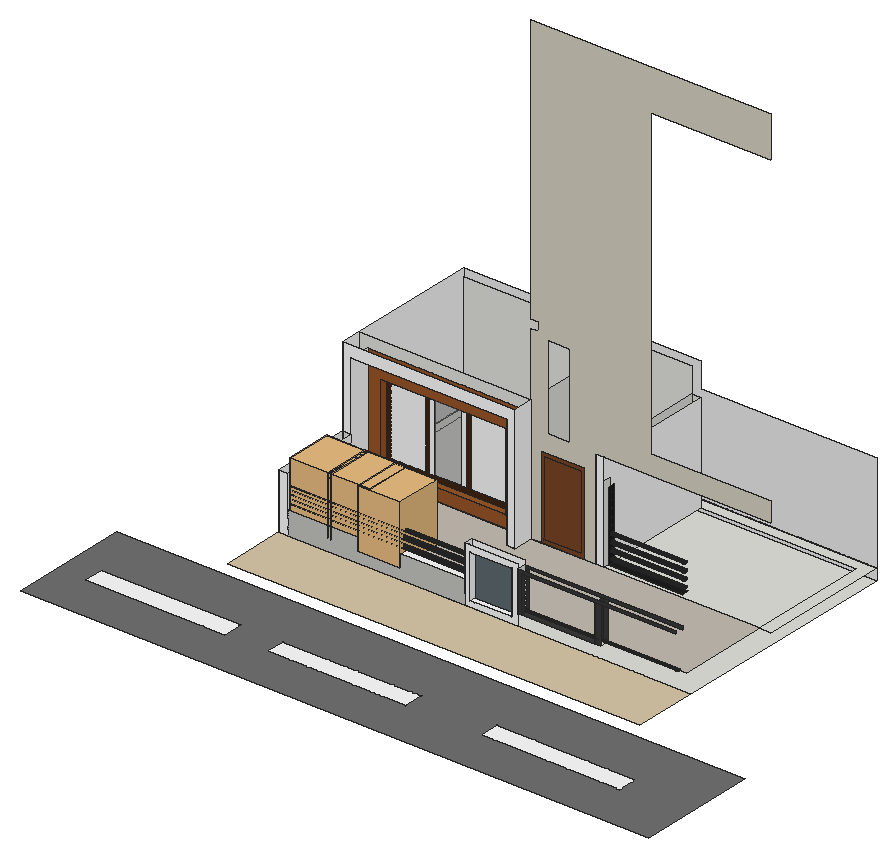
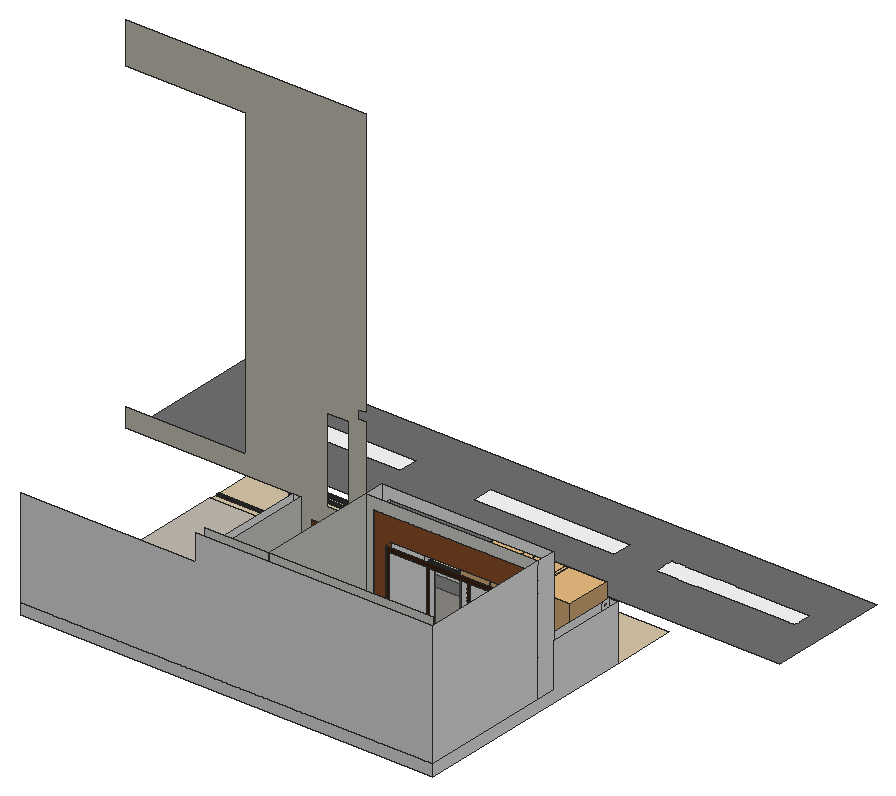
# SketchUp Ruby script. Lengths in inches.
U = 1.inch
M = Sketchup.active_model
def pt(a) = Geom::Point3d.new(a.map { |v| v * U })
def face(e, loops, mat)
  f = e.add_face(loops[0].map { |a| pt(a) })
  loops[1..].each { |l| e.add_face(l.map { |a| pt(a) }).erase! }
  f.material = f.back_material = mat if mat
  f
end
# faces: each face lists its corners as indices into pts; further lists are holes
def faces(e, pts, list, mat = nil) = list.each { |f| face(e, (f[0].is_a?(Array) ? f : [f]).map { |l| l.map { |i| pts[i] } }, mat) }
# xy, xz, yz: faces in a plane at the given z, y or x. An outline is a flat list of corners, or four numbers for a rectangle; further outlines are holes
def ring(l) = l.size == 4 ? [[l[0], l[1]], [l[2], l[1]], [l[2], l[3]], [l[0], l[3]]] : l.each_slice(2).to_a
def flat(e, list, mat, &to3) = list.each { |f| face(e, (f[0].is_a?(Array) ? f : [f]).map { |l| ring(l).map { |u, v| to3.(u, v) } }, mat) }
def xy(e, z, list, mat = nil) = flat(e, list, mat) { |x, y| [x, y, z] }
def xz(e, y, list, mat = nil) = flat(e, list, mat) { |x, z| [x, y, z] }
def yz(e, x, list, mat = nil) = flat(e, list, mat) { |y, z| [x, y, z] }
def lines(e, pts, list) = list.each { |a, b| e.add_line(pt(pts[a]), pt(pts[b])) }
# prism: a flat outline (further loops are holes) pulled along v
def prism(e, loops, v, mat = nil)
  f = face(e, loops, mat); d = Geom::Vector3d.new(v.map { |x| x * U })
  f.pushpull(f.normal.samedirection?(d) ? d.length : -d.length)
end
def box(e, o, s, mat = nil) = prism(e, [[o, [o[0] + s[0], o[1], o[2]], [o[0] + s[0], o[1] + s[1], o[2]], [o[0], o[1] + s[1], o[2]]]], [0, 0, s[2]], mat)
def at(x, y, z, deg = 0) = Geom::Transformation.translation(pt([x, y, z])) * Geom::Transformation.rotation(ORIGIN, Z_AXIS, deg.degrees)
def axes(o, x, y, z) = Geom::Transformation.new([*x, 0, *y, 0, *z, 0, *pt(o).to_a, 1])
def part(name) = M.definitions.add(name)
# library, detail: a bought-in or finely detailed component or shape, given as its bounding box
def library(name, o, s) = part(name).tap { |d| box(d.entities, o, s) }
def detail(e, o, s) = box(e.add_group.entities, o, s)
def put(e, d, t, mat = nil) = e.add_instance(d, t).tap { |i| i.material = mat if mat }
def group(e, t, mat = nil) = e.add_group.tap { |g| g.transformation = t; g.material = mat if mat }.entities
root = M.entities
M.materials.add("[Blinds Vertical Stripe Gray]").color = [247, 247, 247]
M.materials.add("[Carrera Marble]").color = [252, 252, 252]
M.materials.add("[Carrera Marble]1").color = [234, 234, 234]
M.materials.add("[Color M00]").color = [255, 255, 255]
M.materials.add("[Color M05]").color = [114, 114, 114]
M.materials.add("[Color M07]").color = [58, 58, 58]
M.materials.add("[Color M08]").color = [30, 30, 30]
M.materials.add("[Concrete Block 8x8 Gray]").color = [197, 198, 193]
M.materials.add("[Field Rectangle Tile]").color = [196, 189, 179]
M.materials.add("[Field Square Tile]").color = [217, 201, 169]
M.materials.add("[Formica Graystone]").color = [214, 209, 194]
M.materials.add("[Formica Laminate Dark]").color = [50, 53, 60]
M.materials.add("[Formica Speckled Grey]").color = [94, 105, 111]
M.materials.add("[Translucent Glass Gray]").color = [128, 128, 128]
M.materials["[Translucent Glass Gray]"].alpha = 0.5
M.materials.add("[Wood Cherry Original]").color = [152, 86, 42]
M.materials.add("[Wood Veneer 01]").color = [66, 38, 20]
M.materials.add("[Wood Veneer 01]1").color = [120, 70, 37]
c1 = library("chau cay",[-24.34,-109.24,0],[56.46,62.58,79.69])
xy(root,0,[[134.55,270.82,694.52,585.18]])
xy(root,0,[[39.61,61.99,228.17,88.8],[285.48,61.99,474.04,88.8],[576.23,61.99,764.79,88.8]],"[Color M00]")
xy(root,0,[[[0,0,853.75,163.125],[39.61,61.99,228.17,88.8],[285.48,61.99,474.04,88.8],[576.23,61.99,764.79,88.8]]],"[Color M05]")
xy(root,0,[[134.55,183.4,694.52,270.82]],"[Field Square Tile]")
xy(root,7.93,[[394.4,270.82,451.35,278.69]],"[Carrera Marble]")
xy(root,15.1875,[[459.28,270.82,464.36,283.23],[564.04,270.82,571.61,283.23],[134.55,378.85,146.33,406.29],[357.05,378.85,369,406.29],[134.55,406.29,134.55,585.18,694.52,585.18,694.52,406.29,679.23,406.29,679.23,570.65,146.33,570.65,146.33,406.29],
  [146.33,406.29,369,570.65],[369,406.29,456.06,570.65],[456.06,406.29,467.61,570.65]])
xy(root,15.1875,[[464.36,270.82,564.04,283.23]],"[Color M07]")
xy(root,15.1875,[[146.33,283.23,679.23,283.23,679.23,406.29,369,406.29,369,378.85,357.05,378.85,357.05,406.29,146.33,406.29]],"[Field Rectangle Tile]")
xy(root,19.3125,[[473.77,406.29,574.36,416.16]],"[Color M08]")
xy(root,31.3125,[[146.33,270.82,386.47,283.23]],"[Carrera Marble]")
xy(root,31.93,[[163.95,406.29,333.85,416.16]],"[Wood Cherry Original]")
xz(root,270.82,[[134.55,0,146.33,75.25],[[386.47,0,459.28,75.25],[394.4,7.93,451.35,67.32]]],"[Carrera Marble]")
xz(root,270.82,[[459.28,15.1875,464.36,15.1875,464.36,65.34,673.42,65.34,673.42,69.375,459.28,69.375],[564.04,15.1875,571.61,65.34]],"[Color M07]")
xz(root,270.82,[[146.33,0,386.47,31.3125]],"[Concrete Block 8x8 Gray]")
xz(root,278.69,[[394.4,7.93,451.35,67.32]],"[Formica Speckled Grey]")
xz(root,283.23,[[386.47,15.1875,459.28,75.25]],"[Carrera Marble]")
xz(root,283.23,[[459.28,15.1875,459.28,69.375,673.42,69.375,673.42,65.34,464.36,65.34,464.36,15.1875],[564.04,15.1875,571.61,65.34]],"[Color M07]")
xz(root,283.23,[[146.33,15.1875,386.47,31.3125]],"[Concrete Block 8x8 Gray]")
xz(root,378.85,[[134.55,15.1875,146.33,75.25]])
xz(root,378.85,[[357.05,15.1875,369,15.1875,369,183.6875,134.55,183.6875,134.55,75.25,146.33,75.25,146.33,168.73,357.05,168.73]],"[Carrera Marble]")
xz(root,406.29,[[134.55,15.1875,134.55,183.6875,369,183.6875,369,15.1875,357.05,15.1875,357.05,168.73,146.33,168.73,146.33,15.1875]])
xz(root,406.29,[[456.06,15.1875,467.61,149.125]],"[Carrera Marble]")
xz(root,406.29,[[[369,15.1875,381.33,15.1875,381.33,126.53,442.15,126.53,442.15,15.1875,456.06,15.1875,456.06,149.125,694.52,149.125,694.52,175.14,531.06,175.14,531.06,590.25,694.52,590.25,694.52,645.75,369,645.75,369,282.625,378.87,282.625,378.87,270.8125,369,270.8125],[391.83,149.97,420.7,264.27]]],"[Formica Graystone]")
xz(root,406.29,[[[146.33,15.1875,357.05,168.73],[163.95,31.93,333.85,136.93]]],"[Wood Cherry Original]")
xz(root,406.29,[[[381.33,15.1875,442.15,126.53],[386.24,20.1,437.24,121.625]],[386.24,20.1,437.24,121.625]],"[Wood Veneer 01]1")
xz(root,416.16,[[170.57,38.55,217.46,130.31],[223.37,38.55,229.51,130.31],[266.3,38.55,272.95,130.31],[278.86,38.55,327.23,130.31]],"[Blinds Vertical Stripe Gray]")
xz(root,416.16,[[229.51,38.55,266.3,130.31]],"[Translucent Glass Gray]")
xz(root,416.16,[[[163.95,31.93,333.85,136.93],[170.57,38.55,327.23,130.31]],[217.46,38.55,223.37,130.31],[272.95,38.55,278.86,130.31]],"[Wood Veneer 01]")
xz(root,570.65,[[146.33,15.1875,369,183.6875],[369,15.1875,456.06,183.6875],[456.06,15.1875,467.61,149.125]])
xz(root,585.18,[[134.55,0,694.52,15.1875],[134.55,15.1875,134.55,183.6875,456.06,183.6875,456.06,149.125,694.52,149.125,694.52,15.1875]],"[Carrera Marble]1")
yz(root,134.55,[[270.82,0,270.82,75.25,378.85,75.25,378.85,15.1875,585.18,15.1875,585.18,0],[378.85,15.1875,406.29,183.6875],[406.29,15.1875,585.18,183.6875]],"[Carrera Marble]")
yz(root,146.33,[[277.43,35.26,276.8,35.35,276.21,35.59,275.71,35.98,275.32,36.48,275.08,37.07,274.99,37.7,275.08,38.33,275.32,38.92,275.71,39.42,276.21,39.8125,276.8,40.05,277.43,40.14,278.0625,40.05,278.65,39.8125,279.15,39.42,279.54,38.92,279.78,38.33,279.87,37.7,279.78,37.07,279.54,36.48,279.15,35.98,278.65,35.59,278.0625,35.35],[277.43,46.33,276.8,46.41,276.21,46.65,275.71,47.04,275.32,47.54,275.08,48.13,274.99,48.76,275.08,49.39,275.32,49.98,275.71,50.49,276.21,50.875,276.8,51.12,277.43,51.2,278.0625,51.12,278.65,50.875,279.15,50.49,279.54,49.98,279.78,49.39,279.87,48.76,279.78,48.13,279.54,47.54,279.15,47.04,278.65,46.65,278.0625,46.41],[277.43,57.01,276.8,57.1,276.21,57.34,275.71,57.73,275.32,58.23,275.08,58.82,274.99,59.45,275.08,60.08,275.32,60.67,275.71,61.17,276.21,61.5625,276.8,61.8,277.43,61.89,278.0625,61.8,278.65,61.5625,279.15,61.17,279.54,60.67,279.78,60.08,279.87,59.45,279.78,58.82,279.54,58.23,279.15,57.73,278.65,57.34,278.0625,57.1]])
yz(root,146.33,[[283.23,15.1875,378.85,75.25],[378.85,15.1875,406.29,168.73],[[270.82,31.3125,283.23,75.25],[277.43,35.26,276.8,35.35,276.21,35.59,275.71,35.98,275.32,36.48,275.08,37.07,274.99,37.7,275.08,38.33,275.32,38.92,275.71,39.42,276.21,39.8125,276.8,40.05,277.43,40.14,278.0625,40.05,278.65,39.8125,279.15,39.42,279.54,38.92,279.78,38.33,279.87,37.7,279.78,37.07,279.54,36.48,279.15,35.98,278.65,35.59,278.0625,35.35],[277.43,57.01,276.8,57.1,276.21,57.34,275.71,57.73,275.32,58.23,275.08,58.82,274.99,59.45,275.08,60.08,275.32,60.67,275.71,61.17,276.21,61.5625,276.8,61.8,277.43,61.89,278.0625,61.8,278.65,61.5625,279.15,61.17,279.54,60.67,279.78,60.08,279.87,59.45,279.78,58.82,279.54,58.23,279.15,57.73,278.65,57.34,278.0625,57.1],[277.43,46.33,276.8,46.41,276.21,46.65,275.71,47.04,275.32,47.54,275.08,48.13,274.99,48.76,275.08,49.39,275.32,49.98,275.71,50.49,276.21,50.875,276.8,51.12,277.43,51.2,278.0625,51.12,278.65,50.875,279.15,50.49,279.54,49.98,279.78,49.39,279.87,48.76,279.78,48.13,279.54,47.54,279.15,47.04,278.65,46.65,278.0625,46.41],[277.43,67.33,276.8,67.41,276.21,67.65,275.71,68.04,275.32,68.54,275.08,69.13,274.99,69.76,275.08,70.39,275.32,70.98,275.71,71.49,276.21,71.875,276.8,72.12,277.43,72.2,278.0625,72.12,278.65,71.875,279.15,71.49,279.54,70.98,279.78,70.39,279.87,69.76,279.78,69.13,279.54,68.54,279.15,68.04,278.65,67.65,278.0625,67.41]]],"[Carrera Marble]")
yz(root,163.95,[[406.29,31.93,416.16,136.93]],"[Wood Cherry Original]")
yz(root,333.85,[[406.29,31.93,416.16,136.93]],"[Wood Cherry Original]")
yz(root,357.05,[[378.85,15.1875,406.29,168.73]],"[Carrera Marble]")
yz(root,369,[[406.29,15.1875,570.65,183.6875]])
yz(root,369,[[378.85,15.1875,406.29,183.6875]],"[Carrera Marble]")
yz(root,386.47,[[270.82,15.1875,283.23,31.3125]])
yz(root,386.47,[[[270.82,31.3125,283.23,75.25],[277.43,67.33,278.0625,67.41,278.65,67.65,279.15,68.04,279.54,68.54,279.78,69.13,279.87,69.76,279.78,70.39,279.54,70.98,279.15,71.49,278.65,71.875,278.0625,72.12,277.43,72.2,276.8,72.12,276.21,71.875,275.71,71.49,275.32,70.98,275.08,70.39,274.99,69.76,275.08,69.13,275.32,68.54,275.71,68.04,276.21,67.65,276.8,67.41],[277.43,57.01,278.0625,57.1,278.65,57.34,279.15,57.73,279.54,58.23,279.78,58.82,279.87,59.45,279.78,60.08,279.54,60.67,279.15,61.17,278.65,61.5625,278.0625,61.8,277.43,61.89,276.8,61.8,276.21,61.5625,275.71,61.17,275.32,60.67,275.08,60.08,274.99,59.45,275.08,58.82,275.32,58.23,275.71,57.73,276.21,57.34,276.8,57.1],[277.43,46.33,278.0625,46.41,278.65,46.65,279.15,47.04,279.54,47.54,279.78,48.13,279.87,48.76,279.78,49.39,279.54,49.98,279.15,50.49,278.65,50.875,278.0625,51.12,277.43,51.2,276.8,51.12,276.21,50.875,275.71,50.49,275.32,49.98,275.08,49.39,274.99,48.76,275.08,48.13,275.32,47.54,275.71,47.04,276.21,46.65,276.8,46.41],[277.43,35.26,278.0625,35.35,278.65,35.59,279.15,35.98,279.54,36.48,279.78,37.07,279.87,37.7,279.78,38.33,279.54,38.92,279.15,39.42,278.65,39.8125,278.0625,40.05,277.43,40.14,276.8,40.05,276.21,39.8125,275.71,39.42,275.32,38.92,275.08,38.33,274.99,37.7,275.08,37.07,275.32,36.48,275.71,35.98,276.21,35.59,276.8,35.35]]],"[Carrera Marble]")
yz(root,394.4,[[270.82,7.93,278.69,67.32]],"[Carrera Marble]")
yz(root,451.35,[[270.82,7.93,278.69,67.32]],"[Carrera Marble]")
yz(root,456.06,[[406.29,15.1875,570.65,149.125]])
yz(root,459.28,[[270.82,15.1875,283.23,69.375]])
yz(root,464.36,[[276.43,17.77,276.06,17.82,275.71,17.96,275.41,18.1875,275.18,18.49,275.04,18.83,274.99,19.2,275.04,19.58,275.18,19.92,275.41,20.22,275.71,20.45,276.06,20.59,276.43,20.64,276.8,20.59,277.15,20.45,277.44,20.22,277.67,19.92,277.82,19.58,277.87,19.2,277.82,18.83,277.67,18.49,277.44,18.1875,277.15,17.96,276.8,17.82],[276.43,23.27,276.06,23.32,275.71,23.46,275.41,23.6875,275.18,23.99,275.04,24.33,274.99,24.7,275.04,25.08,275.18,25.42,275.41,25.72,275.71,25.95,276.06,26.09,276.43,26.14,276.8,26.09,277.15,25.95,277.44,25.72,277.67,25.42,277.82,25.08,277.87,24.7,277.82,24.33,277.67,23.99,277.44,23.6875,277.15,23.46,276.8,23.32],[276.43,28.77,276.06,28.82,275.71,28.96,275.41,29.1875,275.18,29.49,275.04,29.83,274.99,30.2,275.04,30.58,275.18,30.92,275.41,31.22,275.71,31.45,276.06,31.59,276.43,31.64,276.8,31.59,277.15,31.45,277.44,31.22,277.67,30.92,277.82,30.58,277.87,30.2,277.82,29.83,277.67,29.49,277.44,29.1875,277.15,28.96,276.8,28.82],[276.43,35.2,276.06,35.25,275.71,35.4,275.41,35.625,275.18,35.92,275.04,36.27,274.99,36.64,275.04,37.01,275.18,37.36,275.41,37.66,275.71,37.89,276.06,38.03,276.43,38.08,276.8,38.03,277.15,37.89,277.44,37.66,277.67,37.36,277.82,37.01,277.87,36.64,277.82,36.27,277.67,35.92,277.44,35.625,277.15,35.4,276.8,35.25],[276.43,41.89,276.06,41.94,275.71,42.08,275.41,42.3125,275.18,42.61,275.04,42.96,274.99,43.33,275.04,43.7,275.18,44.05,275.41,44.35,275.71,44.57,276.06,44.72,276.43,44.77,276.8,44.72,277.15,44.57,277.44,44.35,277.67,44.05,277.82,43.7,277.87,43.33,277.82,42.96,277.67,42.61,277.44,42.3125,277.15,42.08,276.8,41.94],
  [276.43,48.08,276.06,48.13,275.71,48.27,275.41,48.5,275.18,48.8,275.04,49.14,274.99,49.52,275.04,49.89,275.18,50.24,275.41,50.53,275.71,50.76,276.06,50.9,276.43,50.95,276.8,50.9,277.15,50.76,277.44,50.53,277.67,50.24,277.82,49.89,277.87,49.52,277.82,49.14,277.67,48.8,277.44,48.5,277.15,48.27,276.8,48.13],[276.43,53.89,276.06,53.94,275.71,54.08,275.41,54.3125,275.18,54.61,275.04,54.96,274.99,55.33,275.04,55.7,275.18,56.05,275.41,56.35,275.71,56.57,276.06,56.72,276.43,56.77,276.8,56.72,277.15,56.57,277.44,56.35,277.67,56.05,277.82,55.7,277.87,55.33,277.82,54.96,277.67,54.61,277.44,54.3125,277.15,54.08,276.8,53.94]])
yz(root,464.36,[[[270.82,15.1875,283.23,65.34],[276.43,17.77,276.06,17.82,275.71,17.96,275.41,18.1875,275.18,18.49,275.04,18.83,274.99,19.2,275.04,19.58,275.18,19.92,275.41,20.22,275.71,20.45,276.06,20.59,276.43,20.64,276.8,20.59,277.15,20.45,277.44,20.22,277.67,19.92,277.82,19.58,277.87,19.2,277.82,18.83,277.67,18.49,277.44,18.1875,277.15,17.96,276.8,17.82],[276.43,23.27,276.06,23.32,275.71,23.46,275.41,23.6875,275.18,23.99,275.04,24.33,274.99,24.7,275.04,25.08,275.18,25.42,275.41,25.72,275.71,25.95,276.06,26.09,276.43,26.14,276.8,26.09,277.15,25.95,277.44,25.72,277.67,25.42,277.82,25.08,277.87,24.7,277.82,24.33,277.67,23.99,277.44,23.6875,277.15,23.46,276.8,23.32],[276.43,48.08,276.06,48.13,275.71,48.27,275.41,48.5,275.18,48.8,275.04,49.14,274.99,49.52,275.04,49.89,275.18,50.24,275.41,50.53,275.71,50.76,276.06,50.9,276.43,50.95,276.8,50.9,277.15,50.76,277.44,50.53,277.67,50.24,277.82,49.89,277.87,49.52,277.82,49.14,277.67,48.8,277.44,48.5,277.15,48.27,276.8,48.13],[276.43,28.77,276.06,28.82,275.71,28.96,275.41,29.1875,275.18,29.49,275.04,29.83,274.99,30.2,275.04,30.58,275.18,30.92,275.41,31.22,275.71,31.45,276.06,31.59,276.43,31.64,276.8,31.59,277.15,31.45,277.44,31.22,277.67,30.92,277.82,30.58,277.87,30.2,277.82,29.83,277.67,29.49,277.44,29.1875,277.15,28.96,276.8,28.82],[276.43,41.89,276.06,41.94,275.71,42.08,275.41,42.3125,275.18,42.61,275.04,42.96,274.99,43.33,275.04,43.7,275.18,44.05,275.41,44.35,275.71,44.57,276.06,44.72,276.43,44.77,276.8,44.72,277.15,44.57,277.44,44.35,277.67,44.05,277.82,43.7,277.87,43.33,277.82,42.96,277.67,42.61,277.44,42.3125,277.15,42.08,276.8,41.94],[276.43,35.2,276.06,35.25,275.71,35.4,275.41,35.625,275.18,35.92,275.04,36.27,274.99,36.64,275.04,37.01,275.18,37.36,275.41,37.66,275.71,37.89,276.06,38.03,276.43,38.08,276.8,38.03,277.15,37.89,277.44,37.66,277.67,37.36,277.82,37.01,277.87,36.64,277.82,36.27,277.67,35.92,277.44,35.625,277.15,35.4,276.8,35.25],[276.43,59.2,276.06,59.25,275.71,59.4,275.41,59.625,275.18,59.92,275.04,60.27,274.99,60.64,275.04,61.01,275.18,61.36,275.41,61.66,275.71,61.89,276.06,62.03,276.43,62.08,276.8,62.03,277.15,61.89,277.44,61.66,277.67,61.36,277.82,61.01,277.87,60.64,277.82,60.27,277.67,59.92,277.44,59.625,277.15,59.4,276.8,59.25],[276.43,53.89,276.06,53.94,275.71,54.08,275.41,54.3125,275.18,54.61,275.04,54.96,274.99,55.33,275.04,55.7,275.18,56.05,275.41,56.35,275.71,56.57,276.06,56.72,276.43,56.77,276.8,56.72,277.15,56.57,277.44,56.35,277.67,56.05,277.82,55.7,277.87,55.33,277.82,54.96,277.67,54.61,277.44,54.3125,277.15,54.08,276.8,53.94]]],"[Color M07]")
yz(root,467.61,[[406.29,15.1875,416.16,119.75]])
yz(root,467.61,[[416.16,15.1875,570.65,15.1875,570.65,149.125,406.29,149.125,406.29,119.75,416.16,119.75]],"[Carrera Marble]")
yz(root,473.77,[[411.5,23.75,411,23.8125,410.53,24.01,410.13,24.32,409.82,24.72,409.63,25.18,409.5625,25.6875,409.63,26.1875,409.82,26.65,410.13,27.06,410.53,27.36,411,27.56,411.5,27.625,412,27.56,412.47,27.36,412.87,27.06,413.18,26.65,413.37,26.1875,413.4375,25.6875,413.37,25.18,413.18,24.72,412.87,24.32,412.47,24.01,412,23.8125],[411.5,33.75,411,33.8125,410.53,34.01,410.13,34.32,409.82,34.72,409.63,35.18,409.5625,35.6875,409.63,36.1875,409.82,36.65,410.13,37.06,410.53,37.36,411,37.56,411.5,37.625,412,37.56,412.47,37.36,412.87,37.06,413.18,36.65,413.37,36.1875,413.4375,35.6875,413.37,35.18,413.18,34.72,412.87,34.32,412.47,34.01,412,33.8125],[411.5,43.75,411,43.8125,410.53,44.01,410.13,44.32,409.82,44.72,409.63,45.18,409.5625,45.6875,409.63,46.1875,409.82,46.65,410.13,47.06,410.53,47.36,411,47.56,411.5,47.625,412,47.56,412.47,47.36,412.87,47.06,413.18,46.65,413.37,46.1875,413.4375,45.6875,413.37,45.18,413.18,44.72,412.87,44.32,412.47,44.01,412,43.8125],[411.5,53.75,411,53.8125,410.53,54.01,410.13,54.32,409.82,54.72,409.63,55.18,409.5625,55.6875,409.63,56.1875,409.82,56.65,410.13,57.06,410.53,57.36,411,57.56,411.5,57.625,412,57.56,412.47,57.36,412.87,57.06,413.18,56.65,413.37,56.1875,413.4375,55.6875,413.37,55.18,413.18,54.72,412.87,54.32,412.47,54.01,412,53.8125]])
yz(root,473.77,[[[406.29,19.3125,416.16,113.6],[411.5,83.75,411,83.8125,410.53,84.01,410.13,84.32,409.82,84.72,409.63,85.18,409.5625,85.6875,409.63,86.1875,409.82,86.65,410.13,87.06,410.53,87.36,411,87.56,411.5,87.625,412,87.56,412.47,87.36,412.87,87.06,413.18,86.65,413.37,86.1875,413.4375,85.6875,413.37,85.18,413.18,84.72,412.87,84.32,412.47,84.01,412,83.8125],[411.5,73.75,411,73.8125,410.53,74.01,410.13,74.32,409.82,74.72,409.63,75.18,409.5625,75.6875,409.63,76.1875,409.82,76.65,410.13,77.06,410.53,77.36,411,77.56,411.5,77.625,412,77.56,412.47,77.36,412.87,77.06,413.18,76.65,413.37,76.1875,413.4375,75.6875,413.37,75.18,413.18,74.72,412.87,74.32,412.47,74.01,412,73.8125],[411.5,63.75,411,63.8125,410.53,64.01,410.13,64.32,409.82,64.72,409.63,65.18,409.5625,65.6875,409.63,66.1875,409.82,66.65,410.13,67.06,410.53,67.36,411,67.56,411.5,67.625,412,67.56,412.47,67.36,412.87,67.06,413.18,66.65,413.37,66.1875,413.4375,65.6875,413.37,65.18,413.18,64.72,412.87,64.32,412.47,64.01,412,63.8125],[411.5,53.75,411,53.8125,410.53,54.01,410.13,54.32,409.82,54.72,409.63,55.18,409.5625,55.6875,409.63,56.1875,409.82,56.65,410.13,57.06,410.53,57.36,411,57.56,411.5,57.625,412,57.56,412.47,57.36,412.87,57.06,413.18,56.65,413.37,56.1875,413.4375,55.6875,413.37,55.18,413.18,54.72,412.87,54.32,412.47,54.01,412,53.8125],[411.5,43.75,411,43.8125,410.53,44.01,410.13,44.32,409.82,44.72,409.63,45.18,409.5625,45.6875,409.63,46.1875,409.82,46.65,410.13,47.06,410.53,47.36,411,47.56,411.5,47.625,412,47.56,412.47,47.36,412.87,47.06,413.18,46.65,413.37,46.1875,413.4375,45.6875,413.37,45.18,413.18,44.72,412.87,44.32,412.47,44.01,412,43.8125],[411.5,33.75,411,33.8125,410.53,34.01,410.13,34.32,409.82,34.72,409.63,35.18,409.5625,35.6875,409.63,36.1875,409.82,36.65,410.13,37.06,410.53,37.36,411,37.56,411.5,37.625,412,37.56,412.47,37.36,412.87,37.06,413.18,36.65,413.37,36.1875,413.4375,35.6875,413.37,35.18,413.18,34.72,412.87,34.32,412.47,34.01,412,33.8125],[411.5,23.75,411,23.8125,410.53,24.01,410.13,24.32,409.82,24.72,409.63,25.18,409.5625,25.6875,409.63,26.1875,409.82,26.65,410.13,27.06,410.53,27.36,411,27.56,411.5,27.625,412,27.56,412.47,27.36,412.87,27.06,413.18,26.65,413.37,26.1875,413.4375,25.6875,413.37,25.18,413.18,24.72,412.87,24.32,412.47,24.01,412,23.8125],[411.5,103.75,411,103.8125,410.53,104.01,410.13,104.32,409.82,104.72,409.63,105.18,409.5625,105.6875,409.63,106.1875,409.82,106.65,410.13,107.06,410.53,107.36,411,107.56,411.5,107.625,412,107.56,412.47,107.36,412.87,107.06,413.18,106.65,413.37,106.1875,413.4375,105.6875,413.37,105.18,413.18,104.72,412.87,104.32,412.47,104.01,412,103.8125],[411.5,93.75,411,93.8125,410.53,94.01,410.13,94.32,409.82,94.72,409.63,95.18,409.5625,95.6875,409.63,96.1875,409.82,96.65,410.13,97.06,410.53,97.36,411,97.56,411.5,97.625,412,97.56,412.47,97.36,412.87,97.06,413.18,96.65,413.37,96.1875,413.4375,95.6875,413.37,95.18,413.18,94.72,412.87,94.32,412.47,94.01,412,93.8125]]],"[Color M08]")
yz(root,564.04,[[270.82,15.1875,283.23,65.34]],"[Color M07]")
p = [[464.36,275.71,17.96],[464.36,276.06,17.82],[673.42,276.06,17.82],[673.42,275.71,17.96],[464.36,276.43,17.77],[673.42,276.43,17.77],
  [464.36,276.8,17.82],[673.42,276.8,17.82],[464.36,277.15,17.96],[673.42,277.15,17.96],[464.36,275.41,18.1875],[673.42,275.41,18.1875],
  [464.36,277.44,18.1875],[673.42,277.44,18.1875],[464.36,275.18,18.49],[673.42,275.18,18.49],[464.36,277.67,18.49],[673.42,277.67,18.49],
  [464.36,275.04,18.83],[673.42,275.04,18.83],[464.36,277.82,18.83],[673.42,277.82,18.83],[464.36,274.99,19.2],[673.42,274.99,19.2],
  [464.36,277.87,19.2],[673.42,277.87,19.2],[464.36,275.04,19.58],[673.42,275.04,19.58],[464.36,277.82,19.58],[673.42,277.82,19.58],
  [473.77,411,23.8125],[473.77,411.5,23.75],[574.36,411.5,23.75],[574.36,411,23.8125],[473.77,412,23.8125],[574.36,412,23.8125],
  [473.77,410.53,24.01],[574.36,410.53,24.01],[473.77,412.47,24.01],[574.36,412.47,24.01],[473.77,410.13,24.32],[574.36,410.13,24.32],
  [473.77,412.87,24.32],[574.36,412.87,24.32],[473.77,409.82,24.72],[574.36,409.82,24.72],[473.77,413.18,24.72],[574.36,413.18,24.72],
  [473.77,409.63,25.18],[574.36,409.63,25.18],[473.77,413.37,25.18],[574.36,413.37,25.18],[473.77,409.5625,25.6875],[574.36,409.5625,25.6875],
  [473.77,413.4375,25.6875],[574.36,413.4375,25.6875],[473.77,409.63,26.1875],[574.36,409.63,26.1875],[473.77,413.37,26.1875],[574.36,413.37,26.1875],
  [473.77,409.82,26.65],[574.36,409.82,26.65],[473.77,413.18,26.65],[574.36,413.18,26.65],[473.77,410.13,27.06],[574.36,410.13,27.06],
  [473.77,412.87,27.06],[574.36,412.87,27.06],[473.77,410.53,27.36],[574.36,410.53,27.36],[473.77,412.47,27.36],[574.36,412.47,27.36],
  [473.77,411,27.56],[574.36,411,27.56],[473.77,412,27.56],[574.36,412,27.56],[473.77,411.5,27.625],[574.36,411.5,27.625],
  [473.77,411,33.8125],[473.77,411.5,33.75],[574.36,411.5,33.75],[574.36,411,33.8125],[473.77,412,33.8125],[574.36,412,33.8125],
  [473.77,410.53,34.01],[574.36,410.53,34.01],[473.77,412.47,34.01],[574.36,412.47,34.01],[473.77,410.13,34.32],[574.36,410.13,34.32],
  [473.77,412.87,34.32],[574.36,412.87,34.32],[473.77,409.82,34.72],[574.36,409.82,34.72],[473.77,413.18,34.72],[574.36,413.18,34.72],
  [473.77,409.63,35.18],[574.36,409.63,35.18],[473.77,413.37,35.18],[574.36,413.37,35.18],[473.77,409.5625,35.6875],[574.36,409.5625,35.6875],
  [473.77,413.4375,35.6875],[574.36,413.4375,35.6875],[146.33,276.21,35.59],[146.33,276.8,35.35],[386.47,276.8,35.35],[386.47,276.21,35.59],
  [146.33,277.43,35.26],[386.47,277.43,35.26],[146.33,278.0625,35.35],[386.47,278.0625,35.35],[146.33,278.65,35.59],[386.47,278.65,35.59],
  [146.33,275.71,35.98],[386.47,275.71,35.98],[146.33,279.15,35.98],[386.47,279.15,35.98],[473.77,409.63,36.1875],[574.36,409.63,36.1875],
  [473.77,413.37,36.1875],[574.36,413.37,36.1875],[146.33,275.32,36.48],[386.47,275.32,36.48],[146.33,279.54,36.48],[386.47,279.54,36.48],
  [473.77,409.82,36.65],[574.36,409.82,36.65],[473.77,413.18,36.65],[574.36,413.18,36.65],[146.33,275.08,37.07],[386.47,275.08,37.07],
  [146.33,279.78,37.07],[386.47,279.78,37.07],[473.77,410.13,37.06],[574.36,410.13,37.06],[473.77,412.87,37.06],[574.36,412.87,37.06],
  [146.33,274.99,37.7],[386.47,274.99,37.7],[146.33,279.87,37.7],[386.47,279.87,37.7],[473.77,410.53,37.36],[574.36,410.53,37.36],
  [473.77,412.47,37.36],[574.36,412.47,37.36],[473.77,411,37.56],[574.36,411,37.56],[473.77,412,37.56],[574.36,412,37.56],
  [473.77,411.5,37.625],[574.36,411.5,37.625],[146.33,275.08,38.33],[386.47,275.08,38.33],[146.33,279.78,38.33],[386.47,279.78,38.33],
  [146.33,275.32,38.92],[386.47,275.32,38.92],[146.33,279.54,38.92],[386.47,279.54,38.92],[146.33,275.71,39.42],[386.47,275.71,39.42],
  [146.33,279.15,39.42],[386.47,279.15,39.42],[146.33,276.21,39.8125],[386.47,276.21,39.8125],[146.33,278.65,39.8125],[386.47,278.65,39.8125],
  [146.33,276.8,40.05],[386.47,276.8,40.05],[146.33,278.0625,40.05],[386.47,278.0625,40.05],[146.33,277.43,40.14],[386.47,277.43,40.14],
  [473.77,411,43.8125],[473.77,411.5,43.75],[574.36,411.5,43.75],[574.36,411,43.8125],[473.77,412,43.8125],[574.36,412,43.8125],
  [473.77,410.53,44.01],[574.36,410.53,44.01],[473.77,412.47,44.01],[574.36,412.47,44.01],[473.77,410.13,44.32],[574.36,410.13,44.32],
  [473.77,412.87,44.32],[574.36,412.87,44.32],[473.77,409.82,44.72],[574.36,409.82,44.72],[473.77,413.18,44.72],[574.36,413.18,44.72],
  [473.77,409.63,45.18],[574.36,409.63,45.18],[473.77,413.37,45.18],[574.36,413.37,45.18],[473.77,409.5625,45.6875],[574.36,409.5625,45.6875],
  [473.77,413.4375,45.6875],[574.36,413.4375,45.6875],[473.77,409.63,46.1875],[574.36,409.63,46.1875],[473.77,413.37,46.1875],[574.36,413.37,46.1875],
  [473.77,409.82,46.65],[574.36,409.82,46.65],[473.77,413.18,46.65],[574.36,413.18,46.65],[146.33,276.8,46.41],[146.33,277.43,46.33],
  [386.47,277.43,46.33],[386.47,276.8,46.41],[146.33,278.0625,46.41],[386.47,278.0625,46.41],[146.33,276.21,46.65],[386.47,276.21,46.65],
  [146.33,278.65,46.65],[386.47,278.65,46.65],[146.33,275.71,47.04],[386.47,275.71,47.04],[146.33,279.15,47.04],[386.47,279.15,47.04],
  [473.77,410.13,47.06],[574.36,410.13,47.06],[473.77,412.87,47.06],[574.36,412.87,47.06],[146.33,275.32,47.54],[386.47,275.32,47.54],
  [146.33,279.54,47.54],[386.47,279.54,47.54],[473.77,410.53,47.36],[574.36,410.53,47.36],[473.77,412.47,47.36],[574.36,412.47,47.36],
  [473.77,411,47.56],[574.36,411,47.56],[473.77,412,47.56],[574.36,412,47.56],[146.33,275.08,48.13],[386.47,275.08,48.13],
  [146.33,279.78,48.13],[386.47,279.78,48.13],[473.77,411.5,47.625],[574.36,411.5,47.625],[146.33,274.99,48.76],[386.47,274.99,48.76],
  [146.33,279.87,48.76],[386.47,279.87,48.76],[146.33,275.08,49.39],[386.47,275.08,49.39],[146.33,279.78,49.39],[386.47,279.78,49.39],
  [146.33,275.32,49.98],[386.47,275.32,49.98],[146.33,279.54,49.98],[386.47,279.54,49.98],[146.33,275.71,50.49],[386.47,275.71,50.49],
  [146.33,279.15,50.49],[386.47,279.15,50.49],[146.33,276.21,50.875],[386.47,276.21,50.875],[146.33,278.65,50.875],[386.47,278.65,50.875],
  [146.33,276.8,51.12],[386.47,276.8,51.12],[146.33,278.0625,51.12],[386.47,278.0625,51.12],[146.33,277.43,51.2],[386.47,277.43,51.2],
  [473.77,411,53.8125],[473.77,411.5,53.75],[574.36,411.5,53.75],[574.36,411,53.8125],[473.77,412,53.8125],[574.36,412,53.8125],
  [473.77,410.53,54.01],[574.36,410.53,54.01],[473.77,412.47,54.01],[574.36,412.47,54.01],[473.77,410.13,54.32],[574.36,410.13,54.32],
  [473.77,412.87,54.32],[574.36,412.87,54.32],[473.77,409.82,54.72],[574.36,409.82,54.72],[473.77,413.18,54.72],[574.36,413.18,54.72],
  [473.77,409.63,55.18],[574.36,409.63,55.18],[473.77,413.37,55.18],[574.36,413.37,55.18],[473.77,409.5625,55.6875],[574.36,409.5625,55.6875],
  [473.77,413.4375,55.6875],[574.36,413.4375,55.6875],[473.77,409.63,56.1875],[574.36,409.63,56.1875],[473.77,413.37,56.1875],[574.36,413.37,56.1875],
  [473.77,409.82,56.65],[574.36,409.82,56.65],[473.77,413.18,56.65],[574.36,413.18,56.65],[473.77,410.13,57.06],[574.36,410.13,57.06],
  [473.77,412.87,57.06],[574.36,412.87,57.06],[146.33,276.8,57.1],[146.33,277.43,57.01],[386.47,277.43,57.01],[386.47,276.8,57.1],
  [146.33,278.0625,57.1],[386.47,278.0625,57.1],[146.33,276.21,57.34],[386.47,276.21,57.34],[146.33,278.65,57.34],[386.47,278.65,57.34],
  [473.77,410.53,57.36],[574.36,410.53,57.36],[473.77,412.47,57.36],[574.36,412.47,57.36],[146.33,275.71,57.73],[386.47,275.71,57.73],
  [146.33,279.15,57.73],[386.47,279.15,57.73],[473.77,411,57.56],[574.36,411,57.56],[473.77,412,57.56],[574.36,412,57.56],
  [473.77,411.5,57.625],[574.36,411.5,57.625],[146.33,275.32,58.23],[386.47,275.32,58.23],[146.33,279.54,58.23],[386.47,279.54,58.23],
  [146.33,275.08,58.82],[386.47,275.08,58.82],[146.33,279.78,58.82],[386.47,279.78,58.82]]
faces(root,p,[[0,1,2,3],[1,4,5,2],[4,6,7,5],[6,8,9,7],[10,0,3,11],[8,12,13,9],[14,10,11,15],[12,16,17,13],
  [18,14,15,19],[16,20,21,17],[22,18,19,23],[20,24,25,21],[26,22,23,27],[24,28,29,25],[104,105,106,107],[105,108,109,106],
  [108,110,111,109],[110,112,113,111],[114,104,107,115],[112,116,117,113],[122,114,115,123],[116,124,125,117],[130,122,123,131],[124,132,133,125],
  [138,130,131,139],[132,140,141,133],[152,138,139,153],[140,154,155,141],[156,152,153,157],[154,158,159,155],[160,156,157,161],[158,162,163,159],
  [164,160,161,165],[162,166,167,163],[168,164,165,169],[166,170,171,167],[172,168,169,173],[170,172,173,171],[208,209,210,211],[209,212,213,210],
  [214,208,211,215],[212,216,217,213],[218,214,215,219],[216,220,221,217],[226,218,219,227],[220,228,229,221],[238,226,227,239],[228,240,241,229],
  [244,238,239,245],[240,246,247,241],[248,244,245,249],[246,250,251,247],[252,248,249,253],[250,254,255,251],[256,252,253,257],[254,258,259,255],
  [260,256,257,261],[258,262,263,259],[264,260,261,265],[262,266,267,263],[268,264,265,269],[266,268,269,267],[308,309,310,311],[309,312,313,310],
  [314,308,311,315],[312,316,317,313],[322,314,315,323],[316,324,325,317],[332,322,323,333],[324,334,335,325],[336,332,333,337],[334,338,339,335]],"[Formica Laminate Dark]")
faces(root,p,[[30,31,32,33],[31,34,35,32],[36,30,33,37],[34,38,39,35],[40,36,37,41],[38,42,43,39],[44,40,41,45],[42,46,47,43],
  [48,44,45,49],[46,50,51,47],[52,48,49,53],[50,54,55,51],[56,52,53,57],[54,58,59,55],[60,56,57,61],[58,62,63,59],
  [64,60,61,65],[62,66,67,63],[68,64,65,69],[66,70,71,67],[72,68,69,73],[70,74,75,71],[76,72,73,77],[74,76,77,75],
  [78,79,80,81],[79,82,83,80],[84,78,81,85],[82,86,87,83],[88,84,85,89],[86,90,91,87],[92,88,89,93],[90,94,95,91],
  [96,92,93,97],[94,98,99,95],[100,96,97,101],[98,102,103,99],[118,100,101,119],[102,120,121,103],[126,118,119,127],[120,128,129,121],
  [134,126,127,135],[128,136,137,129],[142,134,135,143],[136,144,145,137],[146,142,143,147],[144,148,149,145],[150,146,147,151],[148,150,151,149],
  [174,175,176,177],[175,178,179,176],[180,174,177,181],[178,182,183,179],[184,180,181,185],[182,186,187,183],[188,184,185,189],[186,190,191,187],
  [192,188,189,193],[190,194,195,191],[196,192,193,197],[194,198,199,195],[200,196,197,201],[198,202,203,199],[204,200,201,205],[202,206,207,203],
  [222,204,205,223],[206,224,225,207],[230,222,223,231],[224,232,233,225],[234,230,231,235],[232,236,237,233],[242,234,235,243],[236,242,243,237],
  [270,271,272,273],[271,274,275,272],[276,270,273,277],[274,278,279,275],[280,276,277,281],[278,282,283,279],[284,280,281,285],[282,286,287,283],
  [288,284,285,289],[286,290,291,287],[292,288,289,293],[290,294,295,291],[296,292,293,297],[294,298,299,295],[300,296,297,301],[298,302,303,299],
  [304,300,301,305],[302,306,307,303],[318,304,305,319],[306,320,321,307],[326,318,319,327],[320,328,329,321],[330,326,327,331],[328,330,331,329]],"[Color M07]")
put(root,c1,at(172.86,381.03,15.1875))
put(root,c1,at(224.68,381.03,15.1875))
put(root,c1,at(267.01,379.23,15.1875))
